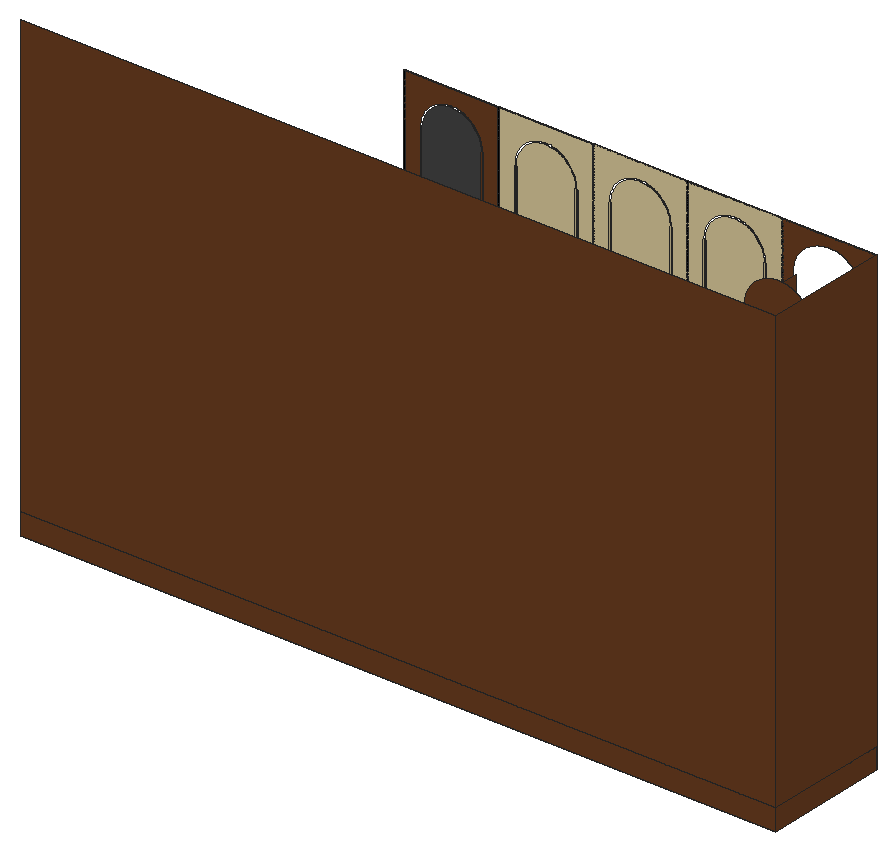
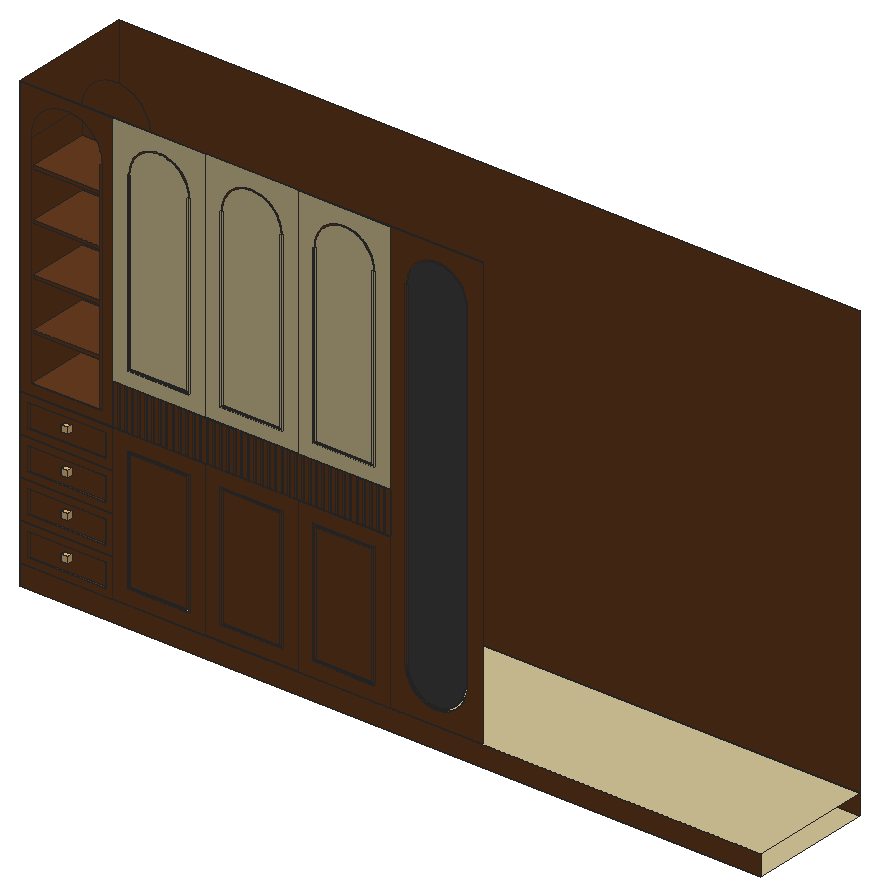
# SketchUp Ruby script. Lengths in inches.
U = 1.inch
M = Sketchup.active_model
def pt(a) = Geom::Point3d.new(a.map { |v| v * U })
def face(e, loops, mat)
  f = e.add_face(loops[0].map { |a| pt(a) })
  loops[1..].each { |l| e.add_face(l.map { |a| pt(a) }).erase! }
  f.material = f.back_material = mat if mat
  f
end
# faces: each face lists its corners as indices into pts; further lists are holes
def faces(e, pts, list, mat = nil) = list.each { |f| face(e, (f[0].is_a?(Array) ? f : [f]).map { |l| l.map { |i| pts[i] } }, mat) }
# xy, xz, yz: faces in a plane at the given z, y or x. An outline is a flat list of corners, or four numbers for a rectangle; further outlines are holes
def ring(l) = l.size == 4 ? [[l[0], l[1]], [l[2], l[1]], [l[2], l[3]], [l[0], l[3]]] : l.each_slice(2).to_a
def flat(e, list, mat, &to3) = list.each { |f| face(e, (f[0].is_a?(Array) ? f : [f]).map { |l| ring(l).map { |u, v| to3.(u, v) } }, mat) }
def xy(e, z, list, mat = nil) = flat(e, list, mat) { |x, y| [x, y, z] }
def xz(e, y, list, mat = nil) = flat(e, list, mat) { |x, z| [x, y, z] }
def yz(e, x, list, mat = nil) = flat(e, list, mat) { |y, z| [x, y, z] }
def lines(e, pts, list) = list.each { |a, b| e.add_line(pt(pts[a]), pt(pts[b])) }
# prism: a flat outline (further loops are holes) pulled along v
def prism(e, loops, v, mat = nil)
  f = face(e, loops, mat); d = Geom::Vector3d.new(v.map { |x| x * U })
  f.pushpull(f.normal.samedirection?(d) ? d.length : -d.length)
end
def box(e, o, s, mat = nil) = prism(e, [[o, [o[0] + s[0], o[1], o[2]], [o[0] + s[0], o[1] + s[1], o[2]], [o[0], o[1] + s[1], o[2]]]], [0, 0, s[2]], mat)
def at(x, y, z, deg = 0) = Geom::Transformation.translation(pt([x, y, z])) * Geom::Transformation.rotation(ORIGIN, Z_AXIS, deg.degrees)
def axes(o, x, y, z) = Geom::Transformation.new([*x, 0, *y, 0, *z, 0, *pt(o).to_a, 1])
def part(name) = M.definitions.add(name)
# library, detail: a bought-in or finely detailed component or shape, given as its bounding box
def library(name, o, s) = part(name).tap { |d| box(d.entities, o, s) }
def detail(e, o, s) = box(e.add_group.entities, o, s)
def put(e, d, t, mat = nil) = e.add_instance(d, t).tap { |i| i.material = mat if mat }
def group(e, t, mat = nil) = e.add_group.tap { |g| g.transformation = t; g.material = mat if mat }.entities
root = M.entities
M.materials.add("138_plaster painted wall texture-seamless").color = [214, 198, 153]
M.materials.add("[0137_Black]").color = [0, 0, 0]
M.materials.add("[Translucent Glass Gray]").color = [66, 66, 66]
M.materials.add("[Wood Veneer 01]").color = [104, 60, 32]
c1 = part("Group\#9")
box(c1.entities,[0,0,0],[14,18,0.6])
c2 = part("Group\#7")
box(c2.entities,[0,0,0],[1,1,8])
c3 = library("Group\#17",[0,0,0],[1.625,1.625,1.31])
xy(root,0,[[24,0,168,24]],"138_plaster painted wall texture-seamless")
xy(root,4,[[24,0,168,24]],"138_plaster painted wall texture-seamless")
xy(root,5.4,[[151.4,23.5,166.6,24]],"[Wood Veneer 01]")
xy(root,7,[[99,24,111,24.2],[117,24,129,24.2],[135,24,147,24.2]],"[Wood Veneer 01]")
xy(root,7.4,[[99.4,24,110.6,24.2],[117.4,24,128.6,24.2],[135.4,24,146.6,24.2]],"[Wood Veneer 01]")
xy(root,10.1,[[151.4,23.5,166.6,24]],"[Wood Veneer 01]")
xy(root,12.9,[[151.4,23.5,166.6,24]],"[Wood Veneer 01]")
xy(root,17.6,[[151.4,23.5,166.6,24]],"[Wood Veneer 01]")
xy(root,20.4,[[151.4,23.5,166.6,24]],"[Wood Veneer 01]")
xy(root,25.1,[[151.4,23.5,166.6,24]],"[Wood Veneer 01]")
xy(root,27.9,[[151.4,23.5,166.6,24]],"[Wood Veneer 01]")
xy(root,30.6,[[99.4,24,110.6,24.2],[117.4,24,128.6,24.2],[135.4,24,146.6,24.2]],"[Wood Veneer 01]")
xy(root,31,[[99,24,111,24.2],[117,24,129,24.2],[135,24,147,24.2]],"[Wood Veneer 01]")
xy(root,32.6,[[151.4,23.5,166.6,24]],"[Wood Veneer 01]")
xy(root,34,[[96,23,114,24],[114,23,132,24],[132,23,150,24]],"138_plaster painted wall texture-seamless")
xy(root,36.4,[[152.4,12,165.6,24.2]],"[Wood Veneer 01]")
xy(root,42,[[96,23,114,24],[114,23,132,24],[132,23,150,24]],"138_plaster painted wall texture-seamless")
xy(root,45,[[99,24,111,24.2],[117,24,129,24.2],[135,24,147,24.2]],"138_plaster painted wall texture-seamless")
xy(root,45.4,[[99.4,24,110.6,24.2],[117.4,24,128.6,24.2],[135.4,24,146.6,24.2]],"138_plaster painted wall texture-seamless")
xz(root,0,[[24,0,168,4],[24,4,168,88]],"[Wood Veneer 01]")
xz(root,12,[[152.4,36.4,152.4,79,152.41,79.38,152.44,79.77,152.5,80.15,152.58,80.52,152.68,80.89,152.8,81.26,152.94,81.61,153.1,81.96,153.28,82.3,153.49,82.625,153.71,82.94,153.94,83.24,154.2,83.53,154.47,83.8,154.76,84.06,155.06,84.29,155.375,84.51,155.7,84.72,156.04,84.9,156.39,85.06,156.74,85.2,157.11,85.32,157.48,85.42,157.85,85.5,158.23,85.56,158.62,85.59,159,85.6,159.38,85.59,159.77,85.56,160.15,85.5,160.52,85.42,160.89,85.32,161.26,85.2,161.61,85.06,161.96,84.9,162.3,84.72,162.625,84.51,162.94,84.29,163.24,84.06,163.53,83.8,163.8,83.53,164.06,83.24,164.29,82.94,164.51,82.625,164.72,82.3,164.9,81.96,165.06,81.61,165.2,81.26,165.32,80.89,165.42,80.52,165.5,80.15,165.56,79.77,165.59,79.38,165.6,79,165.6,36.4]],"[Wood Veneer 01]")
xz(root,23,[[96,34,150,42]],"138_plaster painted wall texture-seamless")
xz(root,23.5,[[151.4,5.4,166.6,10.1],[151.4,12.9,166.6,17.6],[151.4,20.4,166.6,25.1],[151.4,27.9,166.6,32.6]],"[Wood Veneer 01]")
xz(root,24,[[[96.1,42.1,113.9,87.9],[99,45,111,45,111,79,110.99,79.35,110.96,79.7,110.91,80.04,110.84,80.38,110.75,80.72,110.64,81.05,110.51,81.375,110.36,81.69,110.2,82,110.01,82.3,109.8125,82.58,109.6,82.86,109.36,83.12,109.12,83.36,108.86,83.6,108.58,83.8125,108.3,84.01,108,84.2,107.69,84.36,107.375,84.51,107.05,84.64,106.72,84.75,106.38,84.84,106.04,84.91,105.7,84.96,105.35,84.99,105,85,104.65,84.99,104.3,84.96,103.96,84.91,103.62,84.84,103.28,84.75,102.95,84.64,102.625,84.51,102.31,84.36,102,84.2,101.7,84.01,101.42,83.8125,101.14,83.6,100.88,83.36,100.64,83.12,100.4,82.86,100.1875,82.58,99.99,82.3,99.8,82,99.64,81.69,99.49,81.375,99.36,81.05,99.25,80.72,99.16,80.38,99.09,80.04,99.04,79.7,99.01,79.35,99,79]],[[114.1,42.1,131.9,87.9],[117,45,129,45,129,79,128.99,79.35,128.96,79.7,128.91,80.04,128.84,80.38,128.75,80.72,128.64,81.05,128.51,81.375,128.36,81.69,128.2,82,128.01,82.3,127.8125,82.58,127.6,82.86,127.36,83.12,127.12,83.36,126.86,83.6,126.58,83.8125,126.3,84.01,126,84.2,125.69,84.36,125.375,84.51,125.05,84.64,124.72,84.75,124.38,84.84,124.04,84.91,123.7,84.96,123.35,84.99,123,85,122.65,84.99,122.3,84.96,121.96,84.91,121.62,84.84,121.28,84.75,120.95,84.64,120.625,84.51,120.31,84.36,120,84.2,119.7,84.01,119.42,83.8125,119.14,83.6,118.88,83.36,118.64,83.12,118.4,82.86,118.1875,82.58,117.99,82.3,117.8,82,117.64,81.69,117.49,81.375,117.36,81.05,117.25,80.72,117.16,80.38,117.09,80.04,117.04,79.7,117.01,79.35,117,79]],[[132.1,42.1,149.9,87.9],[135,45,147,45,147,79,146.99,79.35,146.96,79.7,146.91,80.04,146.84,80.38,146.75,80.72,146.64,81.05,146.51,81.375,146.36,81.69,146.2,82,146.01,82.3,145.8125,82.58,145.6,82.86,145.36,83.12,145.12,83.36,144.86,83.6,144.58,83.8125,144.3,84.01,144,84.2,143.69,84.36,143.375,84.51,143.05,84.64,142.72,84.75,142.38,84.84,142.04,84.91,141.7,84.96,141.35,84.99,141,85,140.65,84.99,140.3,84.96,139.96,84.91,139.62,84.84,139.28,84.75,138.95,84.64,138.625,84.51,138.31,84.36,138,84.2,137.7,84.01,137.42,83.8125,137.14,83.6,136.88,83.36,136.64,83.12,136.4,82.86,136.1875,82.58,135.99,82.3,135.8,82,135.64,81.69,135.49,81.375,135.36,81.05,135.25,80.72,135.16,80.38,135.09,80.04,135.04,79.7,135.01,79.35,135,79]],[99.4,45.4,99.4,79,99.41,79.33,99.4375,79.65,99.49,79.97,99.55,80.29,99.64,80.61,99.74,80.92,99.86,81.22,100,81.51,100.15,81.8,100.32,82.08,100.51,82.34,100.71,82.6,100.93,82.84,101.16,83.07,101.4,83.29,101.66,83.49,101.92,83.68,102.2,83.85,102.49,84,102.78,84.14,103.08,84.26,103.39,84.36,103.71,84.45,104.03,84.51,104.35,84.5625,104.67,84.59,105,84.6,105.33,84.59,105.65,84.5625,105.97,84.51,106.29,84.45,106.61,84.36,106.92,84.26,107.22,84.14,107.51,84,107.8,83.85,108.08,83.68,108.34,83.49,108.6,83.29,108.84,83.07,109.07,82.84,109.29,82.6,109.49,82.34,109.68,82.08,109.85,81.8,110,81.51,110.14,81.22,110.26,80.92,110.36,80.61,110.45,80.29,110.51,79.97,110.5625,79.65,110.59,79.33,110.6,79,110.6,45.4],[117.4,45.4,117.4,79,117.41,79.33,117.4375,79.65,117.49,79.97,117.55,80.29,117.64,80.61,117.74,80.92,117.86,81.22,118,81.51,118.15,81.8,118.32,82.08,118.51,82.34,118.71,82.6,118.93,82.84,119.16,83.07,119.4,83.29,119.66,83.49,119.92,83.68,120.2,83.85,120.49,84,120.78,84.14,121.08,84.26,121.39,84.36,121.71,84.45,122.03,84.51,122.35,84.5625,122.67,84.59,123,84.6,123.33,84.59,123.65,84.5625,123.97,84.51,124.29,84.45,124.61,84.36,124.92,84.26,125.22,84.14,125.51,84,125.8,83.85,126.08,83.68,126.34,83.49,126.6,83.29,126.84,83.07,127.07,82.84,127.29,82.6,127.49,82.34,127.68,82.08,127.85,81.8,128,81.51,128.14,81.22,128.26,80.92,128.36,80.61,128.45,80.29,128.51,79.97,128.5625,79.65,128.59,79.33,128.6,79,128.6,45.4],
  [135.4,45.4,135.4,79,135.41,79.33,135.4375,79.65,135.49,79.97,135.55,80.29,135.64,80.61,135.74,80.92,135.86,81.22,136,81.51,136.15,81.8,136.32,82.08,136.51,82.34,136.71,82.6,136.93,82.84,137.16,83.07,137.4,83.29,137.66,83.49,137.92,83.68,138.2,83.85,138.49,84,138.78,84.14,139.08,84.26,139.39,84.36,139.71,84.45,140.03,84.51,140.35,84.5625,140.67,84.59,141,84.6,141.33,84.59,141.65,84.5625,141.97,84.51,142.29,84.45,142.61,84.36,142.92,84.26,143.22,84.14,143.51,84,143.8,83.85,144.08,83.68,144.34,83.49,144.6,83.29,144.84,83.07,145.07,82.84,145.29,82.6,145.49,82.34,145.68,82.08,145.85,81.8,146,81.51,146.14,81.22,146.26,80.92,146.36,80.61,146.45,80.29,146.51,79.97,146.5625,79.65,146.59,79.33,146.6,79,146.6,45.4]],"138_plaster painted wall texture-seamless")
xz(root,24,[[[78,4,96,88],[78.1,4.1,95.9,87.9]],[[96,4,114,34],[96.1,4.1,113.9,33.9]],[[114,4,132,34],[114.1,4.1,131.9,33.9]],[[132,4,150,34],[132.1,4.1,149.9,33.9]],[[150,4,168,11.5],[150.1,4.1,167.9,11.4]],
  [[150,11.5,168,19],[150.1,11.6,167.9,18.9]],[[150,19,168,26.5],[150.1,19.1,167.9,26.4]],[[150,26.5,168,34],[150.1,26.6,167.9,33.9]],[[150,34,168,88],[150.1,34.1,167.9,87.9]],[[96,42,114,88],[96.1,42.1,113.9,87.9]],
  [[114,42,132,88],[114.1,42.1,131.9,87.9]],[[132,42,150,88],[132.1,42.1,149.9,87.9]]],"[0137_Black]")
xz(root,24,[[87,7.4,86.67,7.41,86.35,7.4375,86.03,7.49,85.71,7.55,85.39,7.64,85.08,7.74,84.78,7.86,84.49,8,84.2,8.15,83.92,8.32,83.66,8.51,83.4,8.71,83.16,8.93,82.93,9.16,82.71,9.4,82.51,9.66,82.32,9.92,82.15,10.2,82,10.49,81.86,10.78,81.74,11.08,81.64,11.39,81.55,11.71,81.49,12.03,81.4375,12.35,81.41,12.67,81.4,13,81.4,79,81.41,79.33,81.4375,79.65,81.49,79.97,81.55,80.29,81.64,80.61,81.74,80.92,81.86,81.22,82,81.51,82.15,81.8,82.32,82.08,82.51,82.34,82.71,82.6,82.93,82.84,83.16,83.07,83.4,83.29,83.66,83.49,83.92,83.68,84.2,83.85,84.49,84,84.78,84.14,85.08,84.26,85.39,84.36,85.71,84.45,86.03,84.51,86.35,84.5625,86.67,84.59,87,84.6,87.33,84.59,87.65,84.5625,87.97,84.51,88.29,84.45,88.61,84.36,88.92,84.26,89.22,84.14,89.51,84,89.8,83.85,90.08,83.68,90.34,83.49,90.6,83.29,90.84,83.07,91.07,82.84,91.29,82.6,91.49,82.34,91.68,82.08,91.85,81.8,92,81.51,92.14,81.22,92.26,80.92,92.36,80.61,92.45,80.29,92.51,79.97,92.5625,79.65,92.59,79.33,92.6,79,92.6,13,92.59,12.67,92.5625,12.35,92.51,12.03,92.45,11.71,92.36,11.39,92.26,11.08,92.14,10.78,92,10.49,91.85,10.2,91.68,9.92,91.49,9.66,91.29,9.4,91.07,9.16,90.84,8.93,90.6,8.71,90.34,8.51,90.08,8.32,89.8,8.15,89.51,8,89.22,7.86,88.92,7.74,88.61,7.64,88.29,7.55,87.97,7.49,87.65,7.4375,87.33,7.41]],"[Translucent Glass Gray]")
xz(root,24,[[24,0,168,4],[[78.1,4.1,95.9,87.9],[87,7,87.35,7.01,87.7,7.04,88.04,7.09,88.38,7.16,88.72,7.25,89.05,7.36,89.375,7.49,89.69,7.64,90,7.8,90.3,7.99,90.58,8.1875,90.86,8.4,91.12,8.64,91.36,8.88,91.6,9.14,91.8125,9.42,92.01,9.7,92.2,10,92.36,10.31,92.51,10.625,92.64,10.95,92.75,11.28,92.84,11.62,92.91,11.96,92.96,12.3,92.99,12.65,93,13,93,79,92.99,79.35,92.96,79.7,92.91,80.04,92.84,80.38,92.75,80.72,92.64,81.05,92.51,81.375,92.36,81.69,92.2,82,92.01,82.3,91.8125,82.58,91.6,82.86,91.36,83.12,91.12,83.36,90.86,83.6,90.58,83.8125,90.3,84.01,90,84.2,89.69,84.36,89.375,84.51,89.05,84.64,88.72,84.75,88.38,84.84,88.04,84.91,87.7,84.96,87.35,84.99,87,85,86.65,84.99,86.3,84.96,85.96,84.91,85.62,84.84,85.28,84.75,84.95,84.64,84.625,84.51,84.31,84.36,84,84.2,83.7,84.01,83.42,83.8125,83.14,83.6,82.88,83.36,82.64,83.12,82.4,82.86,82.1875,82.58,81.99,82.3,81.8,82,81.64,81.69,81.49,81.375,81.36,81.05,81.25,80.72,81.16,80.38,81.09,80.04,81.04,79.7,81.01,79.35,81,79,81,13,81.01,12.65,81.04,12.3,81.09,11.96,81.16,11.62,81.25,11.28,81.36,10.95,81.49,10.625,81.64,10.31,81.8,10,81.99,9.7,82.1875,9.42,82.4,9.14,82.64,8.88,82.88,8.64,83.14,8.4,83.42,8.1875,83.7,7.99,84,7.8,84.31,7.64,84.625,7.49,84.95,7.36,85.28,7.25,85.62,7.16,85.96,7.09,86.3,7.04,86.65,7.01]],[[96.1,4.1,113.9,33.9],[99,7,111,31]],[[114.1,4.1,131.9,33.9],[117,7,129,31]],[[132.1,4.1,149.9,33.9],[135,7,147,31]],
  [[150.1,4.1,167.9,11.4],[151.4,5.4,166.6,10.1]],[99.4,7.4,110.6,30.6],[117.4,7.4,128.6,30.6],[135.4,7.4,146.6,30.6],[[150.1,11.6,167.9,18.9],[151.4,12.9,166.6,17.6]],
  [[150.1,19.1,167.9,26.4],[151.4,20.4,166.6,25.1]],[[150.1,26.6,167.9,33.9],[151.4,27.9,166.6,32.6]],[[150.1,34.1,167.9,87.9],[152,36,166,36,166,79,165.99,79.41,165.95,79.8125,165.89,80.22,165.8125,80.61,165.71,81.01,165.58,81.39,165.43,81.77,165.26,82.14,165.0625,82.5,164.85,82.85,164.61,83.18,164.36,83.5,164.09,83.8,163.8,84.09,163.5,84.36,163.18,84.61,162.85,84.85,162.5,85.0625,162.14,85.26,161.77,85.43,161.39,85.58,161.01,85.71,160.61,85.8125,160.22,85.89,159.8125,85.95,159.41,85.99,159,86,158.59,85.99,158.1875,85.95,157.78,85.89,157.39,85.8125,156.99,85.71,156.61,85.58,156.23,85.43,155.86,85.26,155.5,85.0625,155.15,84.85,154.82,84.61,154.5,84.36,154.2,84.09,153.91,83.8,153.64,83.5,153.39,83.18,153.15,82.85,152.9375,82.5,152.74,82.14,152.57,81.77,152.42,81.39,152.29,81.01,152.1875,80.61,152.11,80.22,152.05,79.8125,152.01,79.41,152,79]]],"[Wood Veneer 01]")
yz(root,92.6,[[24,13,24.2,79]],"[Wood Veneer 01]")
yz(root,93,[[24,13,24.2,79]],"[Wood Veneer 01]")
yz(root,96,[[23,34,24,42]],"138_plaster painted wall texture-seamless")
yz(root,99,[[24,45,24.2,79]],"138_plaster painted wall texture-seamless")
yz(root,99,[[24,7,24.2,31]],"[Wood Veneer 01]")
yz(root,99.4,[[24,45.4,24.2,79]],"138_plaster painted wall texture-seamless")
yz(root,99.4,[[24,7.4,24.2,30.6]],"[Wood Veneer 01]")
yz(root,110.6,[[24,45.4,24.2,79]],"138_plaster painted wall texture-seamless")
yz(root,110.6,[[24,7.4,24.2,30.6]],"[Wood Veneer 01]")
yz(root,111,[[24,45,24.2,79]],"138_plaster painted wall texture-seamless")
yz(root,111,[[24,7,24.2,31]],"[Wood Veneer 01]")
yz(root,117,[[24,45,24.2,79]],"138_plaster painted wall texture-seamless")
yz(root,117,[[24,7,24.2,31]],"[Wood Veneer 01]")
yz(root,117.4,[[24,45.4,24.2,79]],"138_plaster painted wall texture-seamless")
yz(root,117.4,[[24,7.4,24.2,30.6]],"[Wood Veneer 01]")
yz(root,128.6,[[24,45.4,24.2,79]],"138_plaster painted wall texture-seamless")
yz(root,128.6,[[24,7.4,24.2,30.6]],"[Wood Veneer 01]")
yz(root,129,[[24,45,24.2,79]],"138_plaster painted wall texture-seamless")
yz(root,129,[[24,7,24.2,31]],"[Wood Veneer 01]")
yz(root,135,[[24,45,24.2,79]],"138_plaster painted wall texture-seamless")
yz(root,135,[[24,7,24.2,31]],"[Wood Veneer 01]")
yz(root,135.4,[[24,45.4,24.2,79]],"138_plaster painted wall texture-seamless")
yz(root,135.4,[[24,7.4,24.2,30.6]],"[Wood Veneer 01]")
yz(root,146.6,[[24,45.4,24.2,79]],"138_plaster painted wall texture-seamless")
yz(root,146.6,[[24,7.4,24.2,30.6]],"[Wood Veneer 01]")
yz(root,147,[[24,45,24.2,79]],"138_plaster painted wall texture-seamless")
yz(root,147,[[24,7,24.2,31]],"[Wood Veneer 01]")
yz(root,150,[[23,34,24,42]],"138_plaster painted wall texture-seamless")
yz(root,151.4,[[23.5,5.4,24,10.1],[23.5,12.9,24,17.6],[23.5,20.4,24,25.1],[23.5,27.9,24,32.6]],"[Wood Veneer 01]")
yz(root,152.4,[[12,36.4,24.2,79]],"[Wood Veneer 01]")
yz(root,165.6,[[12,36.4,24.2,79]],"[Wood Veneer 01]")
yz(root,166.6,[[23.5,5.4,24,10.1],[23.5,12.9,24,17.6],[23.5,20.4,24,25.1],[23.5,27.9,24,32.6]],"[Wood Veneer 01]")
yz(root,168,[[0,0,24,4],[0,4,24,88]],"[Wood Veneer 01]")
p = [[86.3,24,7.04],[85.96,24,7.09],[85.96,24.2,7.09],[86.3,24.2,7.04],[86.65,24,7.01],[86.65,24.2,7.01],
  [87,24,7],[87,24.2,7],[87.35,24,7.01],[87.35,24.2,7.01],[87.7,24,7.04],[87.7,24.2,7.04],
  [88.04,24,7.09],[88.04,24.2,7.09],[85.62,24,7.16],[85.62,24.2,7.16],[88.38,24,7.16],[88.38,24.2,7.16],
  [85.28,24,7.25],[85.28,24.2,7.25],[88.72,24,7.25],[88.72,24.2,7.25],[84.95,24,7.36],[84.95,24.2,7.36],
  [89.05,24,7.36],[89.05,24.2,7.36],[84.625,24,7.49],[84.625,24.2,7.49],[86.03,24,7.49],[86.35,24,7.4375],
  [86.35,24.2,7.4375],[86.03,24.2,7.49],[86.67,24,7.41],[86.67,24.2,7.41],[87,24,7.4],[87,24.2,7.4],
  [87.33,24,7.41],[87.33,24.2,7.41],[87.65,24,7.4375],[87.65,24.2,7.4375],[87.97,24,7.49],[87.97,24.2,7.49],
  [89.375,24,7.49],[89.375,24.2,7.49],[84.31,24,7.64],[84.31,24.2,7.64],[85.71,24,7.55],[85.71,24.2,7.55],
  [88.29,24,7.55],[88.29,24.2,7.55],[89.69,24,7.64],[89.69,24.2,7.64],[84,24,7.8],[84,24.2,7.8],
  [85.08,24,7.74],[85.39,24,7.64],[85.39,24.2,7.64],[85.08,24.2,7.74],[88.61,24,7.64],[88.61,24.2,7.64],
  [88.92,24,7.74],[88.92,24.2,7.74],[90,24,7.8],[90,24.2,7.8],[84.78,24,7.86],[84.78,24.2,7.86],
  [89.22,24,7.86],[89.22,24.2,7.86],[83.7,24,7.99],[83.7,24.2,7.99],[90.3,24,7.99],[90.3,24.2,7.99],
  [84.49,24,8],[84.49,24.2,8],[89.51,24,8],[89.51,24.2,8],[83.42,24,8.1875],[83.42,24.2,8.1875],
  [84.2,24,8.15],[84.2,24.2,8.15],[89.8,24,8.15],[89.8,24.2,8.15],[90.58,24,8.1875],[90.58,24.2,8.1875],
  [83.14,24,8.4],[83.14,24.2,8.4],[83.92,24,8.32],[83.92,24.2,8.32],[90.08,24,8.32],[90.08,24.2,8.32],
  [90.86,24,8.4],[90.86,24.2,8.4],[83.66,24,8.51],[83.66,24.2,8.51],[90.34,24,8.51],[90.34,24.2,8.51],
  [82.88,24,8.64],[82.88,24.2,8.64],[91.12,24,8.64],[91.12,24.2,8.64],[83.4,24,8.71],[83.4,24.2,8.71],
  [90.6,24,8.71],[90.6,24.2,8.71],[82.64,24,8.88],[82.64,24.2,8.88],[91.36,24,8.88],[91.36,24.2,8.88],
  [83.16,24,8.93],[83.16,24.2,8.93],[90.84,24,8.93],[90.84,24.2,8.93],[82.4,24,9.14],[82.4,24.2,9.14],
  [82.93,24,9.16],[82.93,24.2,9.16],[91.07,24,9.16],[91.07,24.2,9.16],[91.6,24,9.14],[91.6,24.2,9.14],
  [82.1875,24,9.42],[82.1875,24.2,9.42],[91.8125,24,9.42],[91.8125,24.2,9.42],[82.71,24,9.4],[82.71,24.2,9.4],
  [91.29,24,9.4],[91.29,24.2,9.4],[81.99,24,9.7],[81.99,24.2,9.7],[82.51,24,9.66],[82.51,24.2,9.66],
  [91.49,24,9.66],[91.49,24.2,9.66],[92.01,24,9.7],[92.01,24.2,9.7],[81.8,24,10],[81.8,24.2,10],
  [82.32,24,9.92],[82.32,24.2,9.92],[91.68,24,9.92],[91.68,24.2,9.92],[92.2,24,10],[92.2,24.2,10],
  [82.15,24,10.2],[82.15,24.2,10.2],[91.85,24,10.2],[91.85,24.2,10.2],[81.64,24,10.31],[81.64,24.2,10.31],
  [92.36,24,10.31],[92.36,24.2,10.31],[82,24,10.49],[82,24.2,10.49],[92,24,10.49],[92,24.2,10.49],
  [81.49,24,10.625],[81.49,24.2,10.625],[92.51,24,10.625],[92.51,24.2,10.625],[81.86,24,10.78],[81.86,24.2,10.78],
  [92.14,24,10.78],[92.14,24.2,10.78],[81.36,24,10.95],[81.36,24.2,10.95],[92.64,24,10.95],[92.64,24.2,10.95],
  [81.74,24,11.08],[81.74,24.2,11.08],[92.26,24,11.08],[92.26,24.2,11.08],[92.75,24,11.28],[92.75,24.2,11.28],
  [81.64,24,11.39],[81.64,24.2,11.39],[92.36,24,11.39],[92.36,24.2,11.39],[92.84,24,11.62],[92.84,24.2,11.62],
  [81.55,24,11.71],[81.55,24.2,11.71],[92.45,24,11.71],[92.45,24.2,11.71],[92.91,24,11.96],[92.91,24.2,11.96],
  [81.49,24,12.03],[81.49,24.2,12.03],[92.51,24,12.03],[92.51,24.2,12.03],[81.4375,24,12.35],[81.4375,24.2,12.35],
  [92.5625,24,12.35],[92.5625,24.2,12.35],[92.96,24,12.3],[92.96,24.2,12.3],[92.59,24,12.67],[92.59,24.2,12.67],
  [92.99,24,12.65],[92.99,24.2,12.65],[92.6,24,13],[92.6,24.2,13],[93,24,13],[93,24.2,13]]
faces(root,p,[[0,1,2,3],[4,0,3,5],[6,4,5,7],[8,6,7,9],[10,8,9,11],[12,10,11,13],[1,14,15,2],[16,12,13,17],
  [14,18,19,15],[20,16,17,21],[18,22,23,19],[24,20,21,25],[22,26,27,23],[28,29,30,31],[29,32,33,30],[32,34,35,33],
  [34,36,37,35],[36,38,39,37],[38,40,41,39],[42,24,25,43],[26,44,45,27],[46,28,31,47],[40,48,49,41],[50,42,43,51],
  [44,52,53,45],[54,55,56,57],[55,46,47,56],[48,58,59,49],[58,60,61,59],[62,50,51,63],[64,54,57,65],[60,66,67,61],
  [52,68,69,53],[70,62,63,71],[72,64,65,73],[66,74,75,67],[68,76,77,69],[78,72,73,79],[74,80,81,75],[82,70,71,83],
  [76,84,85,77],[86,78,79,87],[80,88,89,81],[90,82,83,91],[92,86,87,93],[88,94,95,89],[84,96,97,85],[98,90,91,99],
  [100,92,93,101],[94,102,103,95],[96,104,105,97],[106,98,99,107],[108,100,101,109],[102,110,111,103],[104,112,113,105],[114,108,109,115],
  [110,116,117,111],[118,106,107,119],[112,120,121,113],[122,118,119,123],[124,114,115,125],[116,126,127,117],[120,128,129,121],[130,124,125,131],
  [126,132,133,127],[134,122,123,135],[128,136,137,129],[138,130,131,139],[132,140,141,133],[142,134,135,143],[144,138,139,145],[140,146,147,141],
  [136,148,149,137],[150,142,143,151],[152,144,145,153],[146,154,155,147],[148,156,157,149],[158,150,151,159],[160,152,153,161],[154,162,163,155],
  [156,164,165,157],[166,158,159,167],[168,160,161,169],[162,170,171,163],[172,166,167,173],[174,168,169,175],[170,176,177,171],[178,172,173,179],
  [180,174,175,181],[176,182,183,177],[184,178,179,185],[186,180,181,187],[182,188,189,183],[190,186,187,191],[188,192,193,189],[194,184,185,195],
  [192,196,197,193],[198,194,195,199],[196,200,201,197],[202,198,199,203]],"[Wood Veneer 01]")
g1 = group(root,at(152.4,6,44.95),"[Wood Veneer 01]")
put(g1,c1,axes([0,0,9.55],[0.94286,0,0],[0,1,0],[0,0,1]))
put(g1,c1,axes([0,0,28.64],[0.94286,0,0],[0,1,0],[0,0,1]))
put(g1,c1,axes([0,0,0],[0.94286,0,0],[0,1,0],[0,0,1]))
put(g1,c1,axes([0,0,19.09],[0.94286,0,0],[0,1,0],[0,0,1]))
g2 = group(root,at(96,23,34),"[Wood Veneer 01]")
put(g2,c2,at(42.4,0,0))
put(g2,c2,at(37.1,0,0))
put(g2,c2,at(33.125,0,0))
put(g2,c2,at(7.95,0,0))
put(g2,c2,at(38.43,0,0))
put(g2,c2,at(35.78,0,0))
put(g2,c2,at(50.35,0,0))
put(g2,c2,at(49.03,0,0))
put(g2,c2,at(43.73,0,0))
put(g2,c2,at(47.7,0,0))
put(g2,c2,at(39.75,0,0))
put(g2,c2,at(45.05,0,0))
put(g2,c2,at(46.375,0,0))
put(g2,c2,at(41.08,0,0))
put(g2,c2,at(31.8,0,0))
put(g2,c2,at(34.45,0,0))
put(g2,c2,at(51.68,0,0))
put(g2,c2,at(30.48,0,0))
put(g2,c2,at(27.83,0,0))
put(g2,c2,at(9.28,0,0))
put(g2,c2,at(14.58,0,0))
put(g2,c2,at(13.25,0,0))
put(g2,c2,at(18.55,0,0))
put(g2,c2,at(17.23,0,0))
put(g2,c2,at(10.6,0,0))
put(g2,c2,at(22.53,0,0))
put(g2,c2,at(23.85,0,0))
put(g2,c2,at(26.5,0,0))
put(g2,c2,at(21.2,0,0))
put(g2,c2,at(15.9,0,0))
put(g2,c2,at(25.18,0,0))
put(g2,c2,at(11.93,0,0))
put(g2,c2,at(19.875,0,0))
put(g2,c2,at(53,0,0))
put(g2,c2,at(29.15,0,0))
put(g2,c2,at(2.65,0,0))
put(g2,c2,at(3.97,0,0))
put(g2,c2,at(6.625,0,0))
put(g2,c2,at(5.3,0,0))
put(g2,c2,at(1.32,0,0))
put(g2,c2,at(0,0,0))
put(root,c3,axes([158.4375,23.5,23.71],[0.75,0,0],[0,0,-0.75],[0,0.75,0]),"[Wood Veneer 01]")
put(root,c3,axes([158.4375,23.5,31.21],[0.75,0,0],[0,0,-0.75],[0,0.75,0]),"[Wood Veneer 01]")
put(root,c3,axes([158.4375,23.5,8.71],[0.75,0,0],[0,0,-0.75],[0,0.75,0]),"[Wood Veneer 01]")
put(root,c3,axes([158.4375,23.5,16.21],[0.75,0,0],[0,0,-0.75],[0,0.75,0]),"[Wood Veneer 01]")
